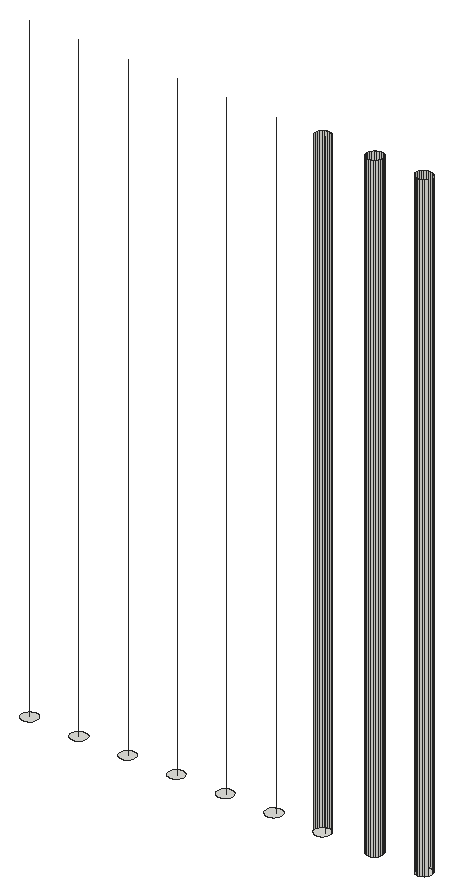
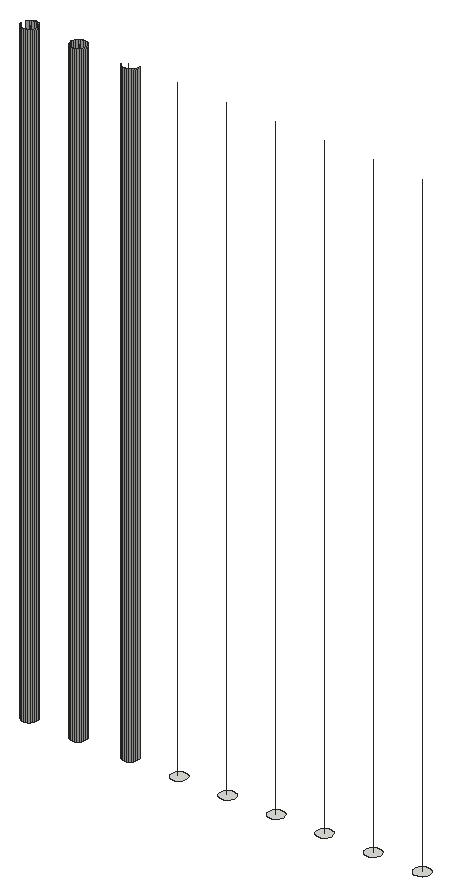
# SketchUp Ruby script. Lengths in inches.
U = 1.inch
M = Sketchup.active_model
def pt(a) = Geom::Point3d.new(a.map { |v| v * U })
def face(e, loops, mat)
  f = e.add_face(loops[0].map { |a| pt(a) })
  loops[1..].each { |l| e.add_face(l.map { |a| pt(a) }).erase! }
  f.material = f.back_material = mat if mat
  f
end
# faces: each face lists its corners as indices into pts; further lists are holes
def faces(e, pts, list, mat = nil) = list.each { |f| face(e, (f[0].is_a?(Array) ? f : [f]).map { |l| l.map { |i| pts[i] } }, mat) }
# xy, xz, yz: faces in a plane at the given z, y or x. An outline is a flat list of corners, or four numbers for a rectangle; further outlines are holes
def ring(l) = l.size == 4 ? [[l[0], l[1]], [l[2], l[1]], [l[2], l[3]], [l[0], l[3]]] : l.each_slice(2).to_a
def flat(e, list, mat, &to3) = list.each { |f| face(e, (f[0].is_a?(Array) ? f : [f]).map { |l| ring(l).map { |u, v| to3.(u, v) } }, mat) }
def xy(e, z, list, mat = nil) = flat(e, list, mat) { |x, y| [x, y, z] }
def xz(e, y, list, mat = nil) = flat(e, list, mat) { |x, z| [x, y, z] }
def yz(e, x, list, mat = nil) = flat(e, list, mat) { |y, z| [x, y, z] }
def lines(e, pts, list) = list.each { |a, b| e.add_line(pt(pts[a]), pt(pts[b])) }
# prism: a flat outline (further loops are holes) pulled along v
def prism(e, loops, v, mat = nil)
  f = face(e, loops, mat); d = Geom::Vector3d.new(v.map { |x| x * U })
  f.pushpull(f.normal.samedirection?(d) ? d.length : -d.length)
end
def box(e, o, s, mat = nil) = prism(e, [[o, [o[0] + s[0], o[1], o[2]], [o[0] + s[0], o[1] + s[1], o[2]], [o[0], o[1] + s[1], o[2]]]], [0, 0, s[2]], mat)
def at(x, y, z, deg = 0) = Geom::Transformation.translation(pt([x, y, z])) * Geom::Transformation.rotation(ORIGIN, Z_AXIS, deg.degrees)
def axes(o, x, y, z) = Geom::Transformation.new([*x, 0, *y, 0, *z, 0, *pt(o).to_a, 1])
def part(name) = M.definitions.add(name)
# library, detail: a bought-in or finely detailed component or shape, given as its bounding box
def library(name, o, s) = part(name).tap { |d| box(d.entities, o, s) }
def detail(e, o, s) = box(e.add_group.entities, o, s)
def put(e, d, t, mat = nil) = e.add_instance(d, t).tap { |i| i.material = mat if mat }
def group(e, t, mat = nil) = e.add_group.tap { |g| g.transformation = t; g.material = mat if mat }.entities
root = M.entities
xy(root,409.875,[[452.36,133.41,452.15,133.44,451.95,133.52,451.78,133.65,451.65,133.82,451.57,134.02,451.54,134.23,451.57,134.4375,451.65,134.63,451.78,134.8,451.95,134.93,452.15,135.01,452.36,135.04,452.57,135.01,452.76,134.93,452.93,134.8,453.06,134.63,453.14,134.4375,453.17,134.23,453.14,134.02,453.06,133.82,452.93,133.65,452.76,133.52,452.57,133.44],[457.67,133.41,457.46,133.44,457.26,133.52,457.09,133.65,456.96,133.82,456.88,134.02,456.86,134.23,456.88,134.4375,456.96,134.63,457.09,134.8,457.26,134.93,457.46,135.01,457.67,135.04,457.88,135.01,458.07,134.93,458.24,134.8,458.37,134.63,458.45,134.4375,458.48,134.23,458.45,134.02,458.37,133.82,458.24,133.65,458.07,133.52,457.88,133.44],[462.92,133.41,462.71,133.44,462.51,133.52,462.34,133.65,462.21,133.82,462.13,134.02,462.11,134.23,462.13,134.4375,462.21,134.63,462.34,134.8,462.51,134.93,462.71,135.01,462.92,135.04,463.13,135.01,463.32,134.93,463.49,134.8,463.62,134.63,463.7,134.4375,463.73,134.23,463.7,134.02,463.62,133.82,463.49,133.65,463.32,133.52,463.13,133.44],[468.17,133.41,467.96,133.44,467.76,133.52,467.59,133.65,467.46,133.82,467.38,134.02,467.36,134.23,467.38,134.4375,467.46,134.63,467.59,134.8,467.76,134.93,467.96,135.01,468.17,135.04,468.38,135.01,468.57,134.93,468.74,134.8,468.87,134.63,468.95,134.4375,468.98,134.23,468.95,134.02,468.87,133.82,468.74,133.65,468.57,133.52,468.38,133.44],[473.42,133.41,473.21,133.44,473.01,133.52,472.84,133.65,472.71,133.82,472.63,134.02,472.61,134.23,472.63,134.4375,472.71,134.63,472.84,134.8,473.01,134.93,473.21,135.01,473.42,135.04,473.63,135.01,473.82,134.93,473.99,134.8,474.12,134.63,474.2,134.4375,474.23,134.23,474.2,134.02,474.12,133.82,473.99,133.65,473.82,133.52,473.63,133.44],
  [478.67,133.41,478.46,133.44,478.26,133.52,478.09,133.65,477.96,133.82,477.88,134.02,477.86,134.23,477.88,134.4375,477.96,134.63,478.09,134.8,478.26,134.93,478.46,135.01,478.67,135.04,478.88,135.01,479.07,134.93,479.24,134.8,479.37,134.63,479.45,134.4375,479.48,134.23,479.45,134.02,479.37,133.82,479.24,133.65,479.07,133.52,478.88,133.44],[483.92,133.41,483.71,133.44,483.51,133.52,483.34,133.65,483.21,133.82,483.13,134.02,483.11,134.23,483.13,134.4375,483.21,134.63,483.34,134.8,483.51,134.93,483.71,135.01,483.92,135.04,484.13,135.01,484.32,134.93,484.49,134.8,484.62,134.63,484.7,134.4375,484.73,134.23,484.7,134.02,484.62,133.82,484.49,133.65,484.32,133.52,484.13,133.44],[489.54,133.41,489.33,133.44,489.14,133.52,488.97,133.65,488.84,133.82,488.76,134.02,488.73,134.23,488.76,134.4375,488.84,134.63,488.97,134.8,489.14,134.93,489.33,135.01,489.54,135.04,489.75,135.01,489.95,134.93,490.12,134.8,490.25,134.63,490.33,134.4375,490.36,134.23,490.33,134.02,490.25,133.82,490.12,133.65,489.95,133.52,489.75,133.44],[494.86,133.41,494.65,133.44,494.45,133.52,494.28,133.65,494.15,133.82,494.07,134.02,494.04,134.23,494.07,134.4375,494.15,134.63,494.28,134.8,494.45,134.93,494.65,135.01,494.86,135.04,495.07,135.01,495.26,134.93,495.43,134.8,495.56,134.63,495.64,134.4375,495.67,134.23,495.64,134.02,495.56,133.82,495.43,133.65,495.26,133.52,495.07,133.44]])
p = [[489.14,133.52,409.875],[489.33,133.44,409.875],[489.33,133.44,477.08],[489.14,133.52,477.08],[489.54,133.41,409.875],[489.54,133.41,477.08],
  [489.75,133.44,409.875],[489.75,133.44,477.08],[489.95,133.52,409.875],[489.95,133.52,477.08],[494.45,133.52,409.875],[494.65,133.44,409.875],
  [494.65,133.44,477.08],[494.45,133.52,477.08],[494.86,133.41,409.875],[494.86,133.41,477.08],[495.07,133.44,409.875],[495.07,133.44,477.08],
  [495.26,133.52,409.875],[495.26,133.52,477.08],[488.97,133.65,409.875],[488.97,133.65,477.08],[490.12,133.65,409.875],[490.12,133.65,477.08],
  [494.28,133.65,409.875],[494.28,133.65,477.08],[495.43,133.65,409.875],[495.43,133.65,477.08],[488.84,133.82,409.875],[488.84,133.82,477.08],
  [490.25,133.82,409.875],[490.25,133.82,477.08],[494.15,133.82,409.875],[494.15,133.82,477.08],[495.56,133.82,409.875],[495.56,133.82,477.08],
  [488.76,134.02,409.875],[488.76,134.02,477.08],[490.33,134.02,409.875],[490.33,134.02,477.08],[494.07,134.02,409.875],[494.07,134.02,477.08],
  [483.11,134.23,409.875],[483.13,134.02,409.875],[483.13,134.02,477.08],[483.11,134.23,477.08],[488.73,134.23,409.875],[488.73,134.23,477.08],
  [490.36,134.23,409.875],[490.36,134.23,477.08],[494.04,134.23,409.875],[494.04,134.23,477.08],[483.13,134.4375,409.875],[483.13,134.4375,477.08],
  [488.76,134.4375,409.875],[488.76,134.4375,477.08],[490.33,134.4375,409.875],[490.33,134.4375,477.08],[494.07,134.4375,409.875],[494.07,134.4375,477.08],
  [483.21,134.63,409.875],[483.21,134.63,477.08],[488.84,134.63,409.875],[488.84,134.63,477.08],[490.25,134.63,409.875],[490.25,134.63,477.08],
  [494.15,134.63,409.875],[494.15,134.63,477.08],[495.64,134.4375,409.875],[495.56,134.63,409.875],[495.56,134.63,477.08],[495.64,134.4375,477.08],
  [483.34,134.8,409.875],[483.34,134.8,477.08],[484.62,134.63,409.875],[484.49,134.8,409.875],[484.49,134.8,477.08],[484.62,134.63,477.08],
  [488.97,134.8,409.875],[488.97,134.8,477.08],[490.12,134.8,409.875],[490.12,134.8,477.08],[494.28,134.8,409.875],[494.28,134.8,477.08],
  [495.43,134.8,409.875],[495.43,134.8,477.08],[483.51,134.93,409.875],[483.51,134.93,477.08],[484.32,134.93,409.875],[484.32,134.93,477.08],
  [489.14,134.93,409.875],[489.14,134.93,477.08],[489.95,134.93,409.875],[489.95,134.93,477.08],[494.45,134.93,409.875],[494.45,134.93,477.08],
  [495.26,134.93,409.875],[495.26,134.93,477.08],[483.71,135.01,409.875],[483.71,135.01,477.08],[484.13,135.01,409.875],[484.13,135.01,477.08],
  [489.33,135.01,409.875],[489.33,135.01,477.08],[489.75,135.01,409.875],[489.75,135.01,477.08],[494.65,135.01,409.875],[494.65,135.01,477.08],
  [495.07,135.01,409.875],[495.07,135.01,477.08],[483.92,135.04,409.875],[483.92,135.04,477.08],[489.54,135.04,409.875],[489.54,135.04,477.08],
  [494.86,135.04,409.875],[494.86,135.04,477.08],[494.82,134.22,477.08],[494.82,134.22,409.875],[489.51,134.22,477.08],[489.51,134.22,409.875],
  [484.2,134.22,477.08],[484.2,134.22,409.875],[478.89,134.22,477.08],[478.89,134.22,409.875],[473.57,134.22,477.08],[473.57,134.22,409.875],
  [468.26,134.22,477.08],[468.26,134.22,409.875],[462.95,134.22,477.08],[462.95,134.22,409.875],[457.64,134.22,477.08],[457.64,134.22,409.875],
  [452.32,134.22,477.08],[452.32,134.22,409.875]]
faces(root,p,[[0,1,2,3],[1,4,5,2],[4,6,7,5],[6,8,9,7],[10,11,12,13],[11,14,15,12],[14,16,17,15],[16,18,19,17],
  [20,0,3,21],[8,22,23,9],[24,10,13,25],[18,26,27,19],[28,20,21,29],[22,30,31,23],[32,24,25,33],[26,34,35,27],
  [36,28,29,37],[30,38,39,31],[40,32,33,41],[42,43,44,45],[46,36,37,47],[38,48,49,39],[50,40,41,51],[52,42,45,53],
  [54,46,47,55],[48,56,57,49],[58,50,51,59],[60,52,53,61],[62,54,55,63],[56,64,65,57],[66,58,59,67],[68,69,70,71],
  [72,60,61,73],[74,75,76,77],[78,62,63,79],[64,80,81,65],[82,66,67,83],[69,84,85,70],[86,72,73,87],[75,88,89,76],
  [90,78,79,91],[80,92,93,81],[94,82,83,95],[84,96,97,85],[98,86,87,99],[88,100,101,89],[102,90,91,103],[92,104,105,93],
  [106,94,95,107],[96,108,109,97],[110,98,99,111],[100,110,111,101],[112,102,103,113],[104,112,113,105],[114,106,107,115],[108,114,115,109]])
lines(root,p,[[116,117],[118,119],[120,121],[122,123],[124,125],[126,127],[128,129],[130,131],[132,133]])
